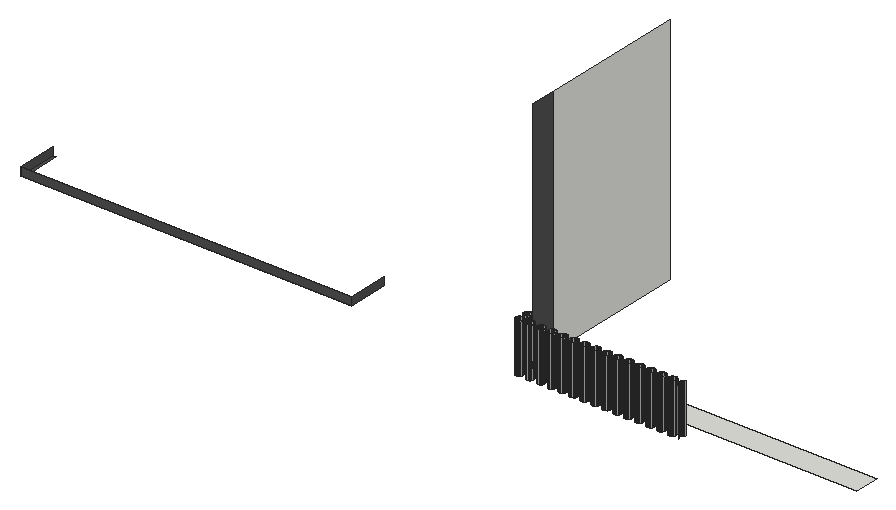
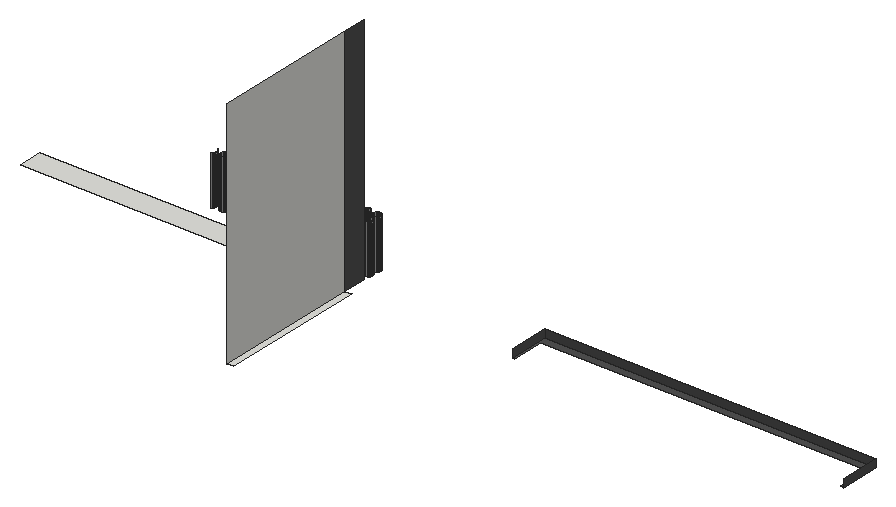
# SketchUp Ruby script. Lengths in inches.
U = 1.inch
M = Sketchup.active_model
def pt(a) = Geom::Point3d.new(a.map { |v| v * U })
def face(e, loops, mat)
  f = e.add_face(loops[0].map { |a| pt(a) })
  loops[1..].each { |l| e.add_face(l.map { |a| pt(a) }).erase! }
  f.material = f.back_material = mat if mat
  f
end
# faces: each face lists its corners as indices into pts; further lists are holes
def faces(e, pts, list, mat = nil) = list.each { |f| face(e, (f[0].is_a?(Array) ? f : [f]).map { |l| l.map { |i| pts[i] } }, mat) }
# xy, xz, yz: faces in a plane at the given z, y or x. An outline is a flat list of corners, or four numbers for a rectangle; further outlines are holes
def ring(l) = l.size == 4 ? [[l[0], l[1]], [l[2], l[1]], [l[2], l[3]], [l[0], l[3]]] : l.each_slice(2).to_a
def flat(e, list, mat, &to3) = list.each { |f| face(e, (f[0].is_a?(Array) ? f : [f]).map { |l| ring(l).map { |u, v| to3.(u, v) } }, mat) }
def xy(e, z, list, mat = nil) = flat(e, list, mat) { |x, y| [x, y, z] }
def xz(e, y, list, mat = nil) = flat(e, list, mat) { |x, z| [x, y, z] }
def yz(e, x, list, mat = nil) = flat(e, list, mat) { |y, z| [x, y, z] }
def lines(e, pts, list) = list.each { |a, b| e.add_line(pt(pts[a]), pt(pts[b])) }
# prism: a flat outline (further loops are holes) pulled along v
def prism(e, loops, v, mat = nil)
  f = face(e, loops, mat); d = Geom::Vector3d.new(v.map { |x| x * U })
  f.pushpull(f.normal.samedirection?(d) ? d.length : -d.length)
end
def box(e, o, s, mat = nil) = prism(e, [[o, [o[0] + s[0], o[1], o[2]], [o[0] + s[0], o[1] + s[1], o[2]], [o[0], o[1] + s[1], o[2]]]], [0, 0, s[2]], mat)
def at(x, y, z, deg = 0) = Geom::Transformation.translation(pt([x, y, z])) * Geom::Transformation.rotation(ORIGIN, Z_AXIS, deg.degrees)
def axes(o, x, y, z) = Geom::Transformation.new([*x, 0, *y, 0, *z, 0, *pt(o).to_a, 1])
def part(name) = M.definitions.add(name)
# library, detail: a bought-in or finely detailed component or shape, given as its bounding box
def library(name, o, s) = part(name).tap { |d| box(d.entities, o, s) }
def detail(e, o, s) = box(e.add_group.entities, o, s)
def put(e, d, t, mat = nil) = e.add_instance(d, t).tap { |i| i.material = mat if mat }
def group(e, t, mat = nil) = e.add_group.tap { |g| g.transformation = t; g.material = mat if mat }.entities
root = M.entities
M.materials.add("[0132_LightGray]").color = [169, 169, 169]
M.materials.add("[0135_DarkGray]").color = [81, 81, 81]
xy(root,180.23,[[54.57,34.6875,54.57,49.6875,55.95,49.6875,55.95,37.6875,176.89,37.6875,176.89,49.6875,177.76,49.6875,177.76,34.6875]],"[0135_DarkGray]")
xy(root,180.28,[[253.31,32.09,252.9375,32.13,252.59,32.28,252.29,32.51,252.0625,32.8,251.92,33.15,251.87,33.52,251.92,33.89,252.0625,34.24,252.29,34.54,252.59,34.77,252.9375,34.91,253.31,34.96,253.68,34.91,254.03,34.77,254.33,34.54,254.55,34.24,254.7,33.89,254.75,33.52,254.7,33.15,254.55,32.8,254.33,32.51,254.03,32.28,253.68,32.13],[257.37,32.09,257,32.13,256.65,32.28,256.35,32.51,256.125,32.8,255.98,33.15,255.93,33.52,255.98,33.89,256.125,34.24,256.35,34.54,256.65,34.77,257,34.91,257.37,34.96,257.74,34.91,258.09,34.77,258.39,34.54,258.62,34.24,258.76,33.89,258.81,33.52,258.76,33.15,258.62,32.8,258.39,32.51,258.09,32.28,257.74,32.13],[261.43,32.09,261.0625,32.13,260.72,32.28,260.42,32.51,260.1875,32.8,260.05,33.15,260,33.52,260.05,33.89,260.1875,34.24,260.42,34.54,260.72,34.77,261.0625,34.91,261.43,34.96,261.81,34.91,262.15,34.77,262.45,34.54,262.68,34.24,262.82,33.89,262.87,33.52,262.82,33.15,262.68,32.8,262.45,32.51,262.15,32.28,261.81,32.13],[265.5,32.09,265.125,32.13,264.78,32.28,264.48,32.51,264.25,32.8,264.11,33.15,264.06,33.52,264.11,33.89,264.25,34.24,264.48,34.54,264.78,34.77,265.125,34.91,265.5,34.96,265.87,34.91,266.22,34.77,266.51,34.54,266.74,34.24,266.88,33.89,266.93,33.52,266.88,33.15,266.74,32.8,266.51,32.51,266.22,32.28,265.87,32.13],[269.56,32.09,269.1875,32.13,268.84,32.28,268.54,32.51,268.3125,32.8,268.17,33.15,268.12,33.52,268.17,33.89,268.3125,34.24,268.54,34.54,268.84,34.77,269.1875,34.91,269.56,34.96,269.93,34.91,270.28,34.77,270.58,34.54,270.8,34.24,270.95,33.89,271,33.52,270.95,33.15,270.8,32.8,270.58,32.51,270.28,32.28,269.93,32.13],
  [273.62,32.09,273.25,32.13,272.9,32.28,272.6,32.51,272.375,32.8,272.23,33.15,272.18,33.52,272.23,33.89,272.375,34.24,272.6,34.54,272.9,34.77,273.25,34.91,273.62,34.96,273.99,34.91,274.34,34.77,274.64,34.54,274.87,34.24,275.01,33.89,275.06,33.52,275.01,33.15,274.87,32.8,274.64,32.51,274.34,32.28,273.99,32.13],[277.68,32.09,277.3125,32.13,276.97,32.28,276.67,32.51,276.4375,32.8,276.3,33.15,276.25,33.52,276.3,33.89,276.4375,34.24,276.67,34.54,276.97,34.77,277.3125,34.91,277.68,34.96,278.06,34.91,278.4,34.77,278.7,34.54,278.93,34.24,279.07,33.89,279.12,33.52,279.07,33.15,278.93,32.8,278.7,32.51,278.4,32.28,278.06,32.13],[281.75,32.09,281.375,32.13,281.03,32.28,280.73,32.51,280.5,32.8,280.36,33.15,280.31,33.52,280.36,33.89,280.5,34.24,280.73,34.54,281.03,34.77,281.375,34.91,281.75,34.96,282.12,34.91,282.47,34.77,282.76,34.54,282.99,34.24,283.13,33.89,283.18,33.52,283.13,33.15,282.99,32.8,282.76,32.51,282.47,32.28,282.12,32.13],[285.81,32.09,285.4375,32.13,285.09,32.28,284.79,32.51,284.5625,32.8,284.42,33.15,284.37,33.52,284.42,33.89,284.5625,34.24,284.79,34.54,285.09,34.77,285.4375,34.91,285.81,34.96,286.18,34.91,286.53,34.77,286.83,34.54,287.05,34.24,287.2,33.89,287.25,33.52,287.2,33.15,287.05,32.8,286.83,32.51,286.53,32.28,286.18,32.13],[289.87,32.09,289.5,32.13,289.15,32.28,288.85,32.51,288.625,32.8,288.48,33.15,288.43,33.52,288.48,33.89,288.625,34.24,288.85,34.54,289.15,34.77,289.5,34.91,289.87,34.96,290.24,34.91,290.59,34.77,290.89,34.54,291.12,34.24,291.26,33.89,291.31,33.52,291.26,33.15,291.12,32.8,290.89,32.51,290.59,32.28,290.24,32.13],
  [293.93,32.09,293.5625,32.13,293.22,32.28,292.92,32.51,292.6875,32.8,292.55,33.15,292.5,33.52,292.55,33.89,292.6875,34.24,292.92,34.54,293.22,34.77,293.5625,34.91,293.93,34.96,294.31,34.91,294.65,34.77,294.95,34.54,295.18,34.24,295.32,33.89,295.37,33.52,295.32,33.15,295.18,32.8,294.95,32.51,294.65,32.28,294.31,32.13],[298,32.09,297.625,32.13,297.28,32.28,296.98,32.51,296.75,32.8,296.61,33.15,296.56,33.52,296.61,33.89,296.75,34.24,296.98,34.54,297.28,34.77,297.625,34.91,298,34.96,298.37,34.91,298.72,34.77,299.01,34.54,299.24,34.24,299.38,33.89,299.43,33.52,299.38,33.15,299.24,32.8,299.01,32.51,298.72,32.28,298.37,32.13],[241.12,35.71,240.75,35.76,240.4,35.9,240.1,36.13,239.875,36.43,239.73,36.78,239.68,37.15,239.73,37.52,239.875,37.87,240.1,38.16,240.4,38.39,240.75,38.54,241.12,38.59,241.49,38.54,241.84,38.39,242.14,38.16,242.37,37.87,242.51,37.52,242.56,37.15,242.51,36.78,242.37,36.43,242.14,36.13,241.84,35.9,241.49,35.76],[240.45,40.6875,360.89,49.6875],[237.76,49.6875,240.45,104.375]])
xz(root,34.6875,[[54.57,180.23,177.76,183.1]],"[0135_DarkGray]")
yz(root,54.57,[[34.6875,180.23,49.6875,183.1]],"[0135_DarkGray]")
yz(root,177.76,[[34.6875,180.23,49.6875,183.1]],"[0135_DarkGray]")
yz(root,240.45,[[49.6875,180.28,104.375,266.7]])
yz(root,240.45,[[40.6875,180.28,49.6875,266.7]],"[0135_DarkGray]")
p = [[240.4,32.28,180.28],[240.75,32.13,180.28],[240.75,32.13,198.6],[240.4,32.28,198.6],[241.12,32.09,180.28],[241.12,32.09,198.6],
  [241.49,32.13,180.28],[241.49,32.13,198.6],[241.84,32.28,180.28],[241.84,32.28,198.6],[244.47,32.28,180.28],[244.8125,32.13,180.28],
  [244.8125,32.13,198.6],[244.47,32.28,198.6],[245.18,32.09,180.28],[245.18,32.09,198.6],[245.56,32.13,180.28],[245.56,32.13,198.6],
  [245.9,32.28,180.28],[245.9,32.28,198.6],[248.53,32.28,180.28],[248.875,32.13,180.28],[248.875,32.13,198.6],[248.53,32.28,198.6],
  [249.25,32.09,180.28],[249.25,32.09,198.6],[249.62,32.13,180.28],[249.62,32.13,198.6],[249.97,32.28,180.28],[249.97,32.28,198.6],
  [252.59,32.28,180.28],[252.9375,32.13,180.28],[252.9375,32.13,198.6],[252.59,32.28,198.6],[253.31,32.09,180.28],[253.31,32.09,198.6],
  [253.68,32.13,180.28],[253.68,32.13,198.6],[254.03,32.28,180.28],[254.03,32.28,198.6],[256.65,32.28,180.28],[257,32.13,180.28],
  [257,32.13,198.6],[256.65,32.28,198.6],[257.37,32.09,180.28],[257.37,32.09,198.6],[257.74,32.13,180.28],[257.74,32.13,198.6],
  [258.09,32.28,180.28],[258.09,32.28,198.6],[260.72,32.28,180.28],[261.0625,32.13,180.28],[261.0625,32.13,198.6],[260.72,32.28,198.6],
  [261.43,32.09,180.28],[261.43,32.09,198.6],[261.81,32.13,180.28],[261.81,32.13,198.6],[262.15,32.28,180.28],[262.15,32.28,198.6],
  [264.78,32.28,180.28],[265.125,32.13,180.28],[265.125,32.13,198.6],[264.78,32.28,198.6],[265.5,32.09,180.28],[265.5,32.09,198.6],
  [265.87,32.13,180.28],[265.87,32.13,198.6],[266.22,32.28,180.28],[266.22,32.28,198.6],[268.84,32.28,180.28],[269.1875,32.13,180.28],
  [269.1875,32.13,198.6],[268.84,32.28,198.6],[269.56,32.09,180.28],[269.56,32.09,198.6],[269.93,32.13,180.28],[269.93,32.13,198.6],
  [270.28,32.28,180.28],[270.28,32.28,198.6],[272.9,32.28,180.28],[273.25,32.13,180.28],[273.25,32.13,198.6],[272.9,32.28,198.6],
  [273.62,32.09,180.28],[273.62,32.09,198.6],[273.99,32.13,180.28],[273.99,32.13,198.6],[274.34,32.28,180.28],[274.34,32.28,198.6],
  [276.97,32.28,180.28],[277.3125,32.13,180.28],[277.3125,32.13,198.6],[276.97,32.28,198.6],[277.68,32.09,180.28],[277.68,32.09,198.6],
  [278.06,32.13,180.28],[278.06,32.13,198.6],[278.4,32.28,180.28],[278.4,32.28,198.6],[281.03,32.28,180.28],[281.375,32.13,180.28],
  [281.375,32.13,198.6],[281.03,32.28,198.6],[281.75,32.09,180.28],[281.75,32.09,198.6],[282.12,32.13,180.28],[282.12,32.13,198.6],
  [282.47,32.28,180.28],[282.47,32.28,198.6],[285.09,32.28,180.28],[285.4375,32.13,180.28],[285.4375,32.13,198.6],[285.09,32.28,198.6],
  [285.81,32.09,180.28],[285.81,32.09,198.6],[286.18,32.13,180.28],[286.18,32.13,198.6],[286.53,32.28,180.28],[286.53,32.28,198.6],
  [289.15,32.28,180.28],[289.5,32.13,180.28],[289.5,32.13,198.6],[289.15,32.28,198.6],[289.87,32.09,180.28],[289.87,32.09,198.6],
  [290.24,32.13,180.28],[290.24,32.13,198.6],[290.59,32.28,180.28],[290.59,32.28,198.6],[293.22,32.28,180.28],[293.5625,32.13,180.28],
  [293.5625,32.13,198.6],[293.22,32.28,198.6],[293.93,32.09,180.28],[293.93,32.09,198.6],[294.31,32.13,180.28],[294.31,32.13,198.6],
  [294.65,32.28,180.28],[294.65,32.28,198.6],[297.28,32.28,180.28],[297.625,32.13,180.28],[297.625,32.13,198.6],[297.28,32.28,198.6],
  [298,32.09,180.28],[298,32.09,198.6],[298.37,32.13,180.28],[298.37,32.13,198.6],[298.72,32.28,180.28],[298.72,32.28,198.6],
  [240.1,32.51,180.28],[240.1,32.51,198.6],[242.14,32.51,180.28],[242.14,32.51,198.6],[244.17,32.51,180.28],[244.17,32.51,198.6],
  [246.2,32.51,180.28],[246.2,32.51,198.6],[248.23,32.51,180.28],[248.23,32.51,198.6],[250.26,32.51,180.28],[250.26,32.51,198.6],
  [252.29,32.51,180.28],[252.29,32.51,198.6],[254.33,32.51,180.28],[254.33,32.51,198.6],[256.35,32.51,180.28],[256.35,32.51,198.6],
  [258.39,32.51,180.28],[258.39,32.51,198.6],[260.42,32.51,180.28],[260.42,32.51,198.6],[262.45,32.51,180.28],[262.45,32.51,198.6],
  [264.48,32.51,180.28],[264.48,32.51,198.6],[266.51,32.51,180.28],[266.51,32.51,198.6],[268.54,32.51,180.28],[268.54,32.51,198.6],
  [270.58,32.51,180.28],[270.58,32.51,198.6],[272.6,32.51,180.28],[272.6,32.51,198.6],[274.64,32.51,180.28],[274.64,32.51,198.6],
  [276.67,32.51,180.28],[276.67,32.51,198.6],[278.7,32.51,180.28],[278.7,32.51,198.6],[280.73,32.51,180.28],[280.73,32.51,198.6],
  [282.76,32.51,180.28],[282.76,32.51,198.6],[284.79,32.51,180.28],[284.79,32.51,198.6],[286.83,32.51,180.28],[286.83,32.51,198.6],
  [288.85,32.51,180.28],[288.85,32.51,198.6],[290.89,32.51,180.28],[290.89,32.51,198.6],[292.92,32.51,180.28],[292.92,32.51,198.6],
  [294.95,32.51,180.28],[294.95,32.51,198.6],[296.98,32.51,180.28],[296.98,32.51,198.6],[299.01,32.51,180.28],[299.01,32.51,198.6],
  [301.04,32.51,180.28],[301.34,32.28,180.28],[301.34,32.28,198.6],[301.04,32.51,198.6],[239.875,32.8,180.28],[239.875,32.8,198.6],
  [242.37,32.8,180.28],[242.37,32.8,198.6],[243.9375,32.8,180.28],[243.9375,32.8,198.6],[246.43,32.8,180.28],[246.43,32.8,198.6],
  [248,32.8,180.28],[248,32.8,198.6],[250.49,32.8,180.28],[250.49,32.8,198.6],[252.0625,32.8,180.28],[252.0625,32.8,198.6],
  [254.55,32.8,180.28],[254.55,32.8,198.6],[256.125,32.8,180.28],[256.125,32.8,198.6],[258.62,32.8,180.28],[258.62,32.8,198.6],
  [260.1875,32.8,180.28],[260.1875,32.8,198.6],[262.68,32.8,180.28],[262.68,32.8,198.6],[264.25,32.8,180.28],[264.25,32.8,198.6],
  [266.74,32.8,180.28],[266.74,32.8,198.6],[268.3125,32.8,180.28],[268.3125,32.8,198.6],[270.8,32.8,180.28],[270.8,32.8,198.6],
  [272.375,32.8,180.28],[272.375,32.8,198.6],[274.87,32.8,180.28],[274.87,32.8,198.6],[276.4375,32.8,180.28],[276.4375,32.8,198.6],
  [278.93,32.8,180.28],[278.93,32.8,198.6],[280.5,32.8,180.28],[280.5,32.8,198.6],[282.99,32.8,180.28],[282.99,32.8,198.6],
  [284.5625,32.8,180.28],[284.5625,32.8,198.6],[287.05,32.8,180.28],[287.05,32.8,198.6],[288.625,32.8,180.28],[288.625,32.8,198.6],
  [291.12,32.8,180.28],[291.12,32.8,198.6],[292.6875,32.8,180.28],[292.6875,32.8,198.6],[295.18,32.8,180.28],[295.18,32.8,198.6],
  [296.75,32.8,180.28],[296.75,32.8,198.6],[299.24,32.8,180.28],[299.24,32.8,198.6],[300.8125,32.8,180.28],[300.8125,32.8,198.6],
  [239.73,33.15,180.28],[239.73,33.15,198.6],[242.51,33.15,180.28],[242.51,33.15,198.6],[243.8,33.15,180.28],[243.8,33.15,198.6],
  [246.57,33.15,180.28],[246.57,33.15,198.6],[247.86,33.15,180.28],[247.86,33.15,198.6],[250.63,33.15,180.28],[250.63,33.15,198.6],
  [251.92,33.15,180.28],[251.92,33.15,198.6],[254.7,33.15,180.28],[254.7,33.15,198.6],[255.98,33.15,180.28],[255.98,33.15,198.6],
  [258.76,33.15,180.28],[258.76,33.15,198.6],[260.05,33.15,180.28],[260.05,33.15,198.6],[262.82,33.15,180.28],[262.82,33.15,198.6],
  [264.11,33.15,180.28],[264.11,33.15,198.6],[266.88,33.15,180.28],[266.88,33.15,198.6],[268.17,33.15,180.28],[268.17,33.15,198.6],
  [270.95,33.15,180.28],[270.95,33.15,198.6],[272.23,33.15,180.28],[272.23,33.15,198.6],[275.01,33.15,180.28],[275.01,33.15,198.6],
  [276.3,33.15,180.28],[276.3,33.15,198.6],[279.07,33.15,180.28],[279.07,33.15,198.6],[280.36,33.15,180.28],[280.36,33.15,198.6],
  [283.13,33.15,180.28],[283.13,33.15,198.6],[284.42,33.15,180.28],[284.42,33.15,198.6],[287.2,33.15,180.28],[287.2,33.15,198.6],
  [288.48,33.15,180.28],[288.48,33.15,198.6],[291.26,33.15,180.28],[291.26,33.15,198.6],[292.55,33.15,180.28],[292.55,33.15,198.6],
  [295.32,33.15,180.28],[295.32,33.15,198.6],[296.61,33.15,180.28],[296.61,33.15,198.6],[299.38,33.15,180.28],[299.38,33.15,198.6],
  [300.67,33.15,180.28],[300.67,33.15,198.6],[239.68,33.52,180.28],[239.68,33.52,198.6],[242.56,33.52,180.28],[242.56,33.52,198.6],
  [243.75,33.52,180.28],[243.75,33.52,198.6],[246.62,33.52,180.28],[246.62,33.52,198.6],[247.81,33.52,180.28],[247.81,33.52,198.6],
  [250.68,33.52,180.28],[250.68,33.52,198.6],[251.87,33.52,180.28],[251.87,33.52,198.6],[254.75,33.52,180.28],[254.75,33.52,198.6],
  [255.93,33.52,180.28],[255.93,33.52,198.6],[258.81,33.52,180.28],[258.81,33.52,198.6],[260,33.52,180.28],[260,33.52,198.6],
  [262.87,33.52,180.28],[262.87,33.52,198.6],[264.06,33.52,180.28],[264.06,33.52,198.6],[266.93,33.52,180.28],[266.93,33.52,198.6],
  [268.12,33.52,180.28],[268.12,33.52,198.6],[271,33.52,180.28],[271,33.52,198.6],[272.18,33.52,180.28],[272.18,33.52,198.6],
  [275.06,33.52,180.28],[275.06,33.52,198.6],[276.25,33.52,180.28],[276.25,33.52,198.6],[279.12,33.52,180.28],[279.12,33.52,198.6],
  [280.31,33.52,180.28],[280.31,33.52,198.6],[283.18,33.52,180.28],[283.18,33.52,198.6],[284.37,33.52,180.28],[284.37,33.52,198.6],
  [287.25,33.52,180.28],[287.25,33.52,198.6],[288.43,33.52,180.28],[288.43,33.52,198.6],[291.31,33.52,180.28],[291.31,33.52,198.6],
  [292.5,33.52,180.28],[292.5,33.52,198.6],[295.37,33.52,180.28],[295.37,33.52,198.6],[296.56,33.52,180.28],[296.56,33.52,198.6],
  [299.43,33.52,180.28],[299.43,33.52,198.6],[300.62,33.52,180.28],[300.62,33.52,198.6],[239.73,33.89,180.28],[239.73,33.89,198.6],
  [242.51,33.89,180.28],[242.51,33.89,198.6],[243.8,33.89,180.28],[243.8,33.89,198.6],[246.57,33.89,180.28],[246.57,33.89,198.6],
  [247.86,33.89,180.28],[247.86,33.89,198.6],[250.63,33.89,180.28],[250.63,33.89,198.6],[251.92,33.89,180.28],[251.92,33.89,198.6],
  [254.7,33.89,180.28],[254.7,33.89,198.6],[255.98,33.89,180.28],[255.98,33.89,198.6],[258.76,33.89,180.28],[258.76,33.89,198.6],
  [260.05,33.89,180.28],[260.05,33.89,198.6],[262.82,33.89,180.28],[262.82,33.89,198.6],[264.11,33.89,180.28],[264.11,33.89,198.6],
  [266.88,33.89,180.28],[266.88,33.89,198.6],[268.17,33.89,180.28],[268.17,33.89,198.6],[270.95,33.89,180.28],[270.95,33.89,198.6],
  [272.23,33.89,180.28],[272.23,33.89,198.6],[275.01,33.89,180.28],[275.01,33.89,198.6],[276.3,33.89,180.28],[276.3,33.89,198.6],
  [279.07,33.89,180.28],[279.07,33.89,198.6],[280.36,33.89,180.28],[280.36,33.89,198.6],[283.13,33.89,180.28],[283.13,33.89,198.6],
  [284.42,33.89,180.28],[284.42,33.89,198.6],[287.2,33.89,180.28],[287.2,33.89,198.6],[288.48,33.89,180.28],[288.48,33.89,198.6],
  [291.26,33.89,180.28],[291.26,33.89,198.6],[292.55,33.89,180.28],[292.55,33.89,198.6],[295.32,33.89,180.28],[295.32,33.89,198.6],
  [296.61,33.89,180.28],[296.61,33.89,198.6],[299.38,33.89,180.28],[299.38,33.89,198.6],[300.67,33.89,180.28],[300.67,33.89,198.6],
  [239.875,34.24,180.28],[239.875,34.24,198.6],[242.37,34.24,180.28],[242.37,34.24,198.6],[243.9375,34.24,180.28],[243.9375,34.24,198.6],
  [246.43,34.24,180.28],[246.43,34.24,198.6],[248,34.24,180.28],[248,34.24,198.6],[250.49,34.24,180.28],[250.49,34.24,198.6],
  [252.0625,34.24,180.28],[252.0625,34.24,198.6],[254.55,34.24,180.28],[254.55,34.24,198.6],[256.125,34.24,180.28],[256.125,34.24,198.6],
  [258.62,34.24,180.28],[258.62,34.24,198.6],[260.1875,34.24,180.28],[260.1875,34.24,198.6],[262.68,34.24,180.28],[262.68,34.24,198.6],
  [264.25,34.24,180.28],[264.25,34.24,198.6],[266.74,34.24,180.28],[266.74,34.24,198.6],[268.3125,34.24,180.28],[268.3125,34.24,198.6],
  [270.8,34.24,180.28],[270.8,34.24,198.6],[272.375,34.24,180.28],[272.375,34.24,198.6],[274.87,34.24,180.28],[274.87,34.24,198.6],
  [276.4375,34.24,180.28],[276.4375,34.24,198.6],[278.93,34.24,180.28],[278.93,34.24,198.6],[280.5,34.24,180.28],[280.5,34.24,198.6],
  [282.99,34.24,180.28],[282.99,34.24,198.6],[284.5625,34.24,180.28],[284.5625,34.24,198.6],[287.05,34.24,180.28],[287.05,34.24,198.6],
  [288.625,34.24,180.28],[288.625,34.24,198.6],[291.12,34.24,180.28],[291.12,34.24,198.6],[292.6875,34.24,180.28],[292.6875,34.24,198.6],
  [295.18,34.24,180.28],[295.18,34.24,198.6],[296.75,34.24,180.28],[296.75,34.24,198.6],[299.24,34.24,180.28],[299.24,34.24,198.6],
  [300.8125,34.24,180.28],[300.8125,34.24,198.6],[240.1,34.54,180.28],[240.1,34.54,198.6],[242.14,34.54,180.28],[242.14,34.54,198.6],
  [244.17,34.54,180.28],[244.17,34.54,198.6],[246.2,34.54,180.28],[246.2,34.54,198.6],[248.23,34.54,180.28],[248.23,34.54,198.6],
  [250.26,34.54,180.28],[250.26,34.54,198.6],[252.29,34.54,180.28],[252.29,34.54,198.6],[254.33,34.54,180.28],[254.33,34.54,198.6],
  [256.35,34.54,180.28],[256.35,34.54,198.6],[258.39,34.54,180.28],[258.39,34.54,198.6],[260.42,34.54,180.28],[260.42,34.54,198.6],
  [262.45,34.54,180.28],[262.45,34.54,198.6],[264.48,34.54,180.28],[264.48,34.54,198.6],[266.51,34.54,180.28],[266.51,34.54,198.6],
  [268.54,34.54,180.28],[268.54,34.54,198.6],[270.58,34.54,180.28],[270.58,34.54,198.6],[272.6,34.54,180.28],[272.6,34.54,198.6],
  [274.64,34.54,180.28],[274.64,34.54,198.6],[276.67,34.54,180.28],[276.67,34.54,198.6],[278.7,34.54,180.28],[278.7,34.54,198.6],
  [280.73,34.54,180.28],[280.73,34.54,198.6],[282.76,34.54,180.28],[282.76,34.54,198.6],[284.79,34.54,180.28],[284.79,34.54,198.6],
  [286.83,34.54,180.28],[286.83,34.54,198.6],[288.85,34.54,180.28],[288.85,34.54,198.6],[290.89,34.54,180.28],[290.89,34.54,198.6],
  [292.92,34.54,180.28],[292.92,34.54,198.6],[294.95,34.54,180.28],[294.95,34.54,198.6],[296.98,34.54,180.28],[296.98,34.54,198.6],
  [299.01,34.54,180.28],[299.01,34.54,198.6],[301.04,34.54,180.28],[301.04,34.54,198.6],[240.4,34.77,180.28],[240.4,34.77,198.6],
  [241.84,34.77,180.28],[241.84,34.77,198.6],[244.47,34.77,180.28],[244.47,34.77,198.6],[245.9,34.77,180.28],[245.9,34.77,198.6],
  [248.53,34.77,180.28],[248.53,34.77,198.6],[249.97,34.77,180.28],[249.97,34.77,198.6],[252.59,34.77,180.28],[252.59,34.77,198.6],
  [254.03,34.77,180.28],[254.03,34.77,198.6],[256.65,34.77,180.28],[256.65,34.77,198.6],[258.09,34.77,180.28],[258.09,34.77,198.6],
  [260.72,34.77,180.28],[260.72,34.77,198.6],[262.15,34.77,180.28],[262.15,34.77,198.6],[264.78,34.77,180.28],[264.78,34.77,198.6],
  [266.22,34.77,180.28],[266.22,34.77,198.6],[268.84,34.77,180.28],[268.84,34.77,198.6],[270.28,34.77,180.28],[270.28,34.77,198.6],
  [272.9,34.77,180.28],[272.9,34.77,198.6],[274.34,34.77,180.28],[274.34,34.77,198.6],[276.97,34.77,180.28],[276.97,34.77,198.6],
  [278.4,34.77,180.28],[278.4,34.77,198.6],[281.03,34.77,180.28],[281.03,34.77,198.6],[282.47,34.77,180.28],[282.47,34.77,198.6],
  [285.09,34.77,180.28],[285.09,34.77,198.6],[286.53,34.77,180.28],[286.53,34.77,198.6],[289.15,34.77,180.28],[289.15,34.77,198.6],
  [290.59,34.77,180.28],[290.59,34.77,198.6],[293.22,34.77,180.28],[293.22,34.77,198.6],[294.65,34.77,180.28],[294.65,34.77,198.6],
  [297.28,34.77,180.28],[297.28,34.77,198.6],[298.72,34.77,180.28],[298.72,34.77,198.6],[301.34,34.77,180.28],[301.34,34.77,198.6],
  [240.75,34.91,180.28],[240.75,34.91,198.6],[241.49,34.91,180.28],[241.49,34.91,198.6],[244.8125,34.91,180.28],[244.8125,34.91,198.6],
  [245.56,34.91,180.28],[245.56,34.91,198.6],[248.875,34.91,180.28],[248.875,34.91,198.6],[249.62,34.91,180.28],[249.62,34.91,198.6],
  [252.9375,34.91,180.28],[252.9375,34.91,198.6],[253.68,34.91,180.28],[253.68,34.91,198.6],[257,34.91,180.28],[257,34.91,198.6],
  [257.74,34.91,180.28],[257.74,34.91,198.6],[261.0625,34.91,180.28],[261.0625,34.91,198.6],[261.81,34.91,180.28],[261.81,34.91,198.6],
  [265.125,34.91,180.28],[265.125,34.91,198.6],[265.87,34.91,180.28],[265.87,34.91,198.6],[269.1875,34.91,180.28],[269.1875,34.91,198.6],
  [269.93,34.91,180.28],[269.93,34.91,198.6],[273.25,34.91,180.28],[273.25,34.91,198.6],[273.99,34.91,180.28],[273.99,34.91,198.6],
  [277.3125,34.91,180.28],[277.3125,34.91,198.6],[278.06,34.91,180.28],[278.06,34.91,198.6],[281.375,34.91,180.28],[281.375,34.91,198.6],
  [282.12,34.91,180.28],[282.12,34.91,198.6],[285.4375,34.91,180.28],[285.4375,34.91,198.6],[286.18,34.91,180.28],[286.18,34.91,198.6],
  [289.5,34.91,180.28],[289.5,34.91,198.6],[290.24,34.91,180.28],[290.24,34.91,198.6],[293.5625,34.91,180.28],[293.5625,34.91,198.6],
  [294.31,34.91,180.28],[294.31,34.91,198.6],[297.625,34.91,180.28],[297.625,34.91,198.6],[298.37,34.91,180.28],[298.37,34.91,198.6],
  [301.6875,34.91,180.28],[301.6875,34.91,198.6],[241.12,34.96,180.28],[241.12,34.96,198.6],[245.18,34.96,180.28],[245.18,34.96,198.6],
  [249.25,34.96,180.28],[249.25,34.96,198.6],[253.31,34.96,180.28],[253.31,34.96,198.6],[257.37,34.96,180.28],[257.37,34.96,198.6],
  [261.43,34.96,180.28],[261.43,34.96,198.6],[265.5,34.96,180.28],[265.5,34.96,198.6],[269.56,34.96,180.28],[269.56,34.96,198.6],
  [273.62,34.96,180.28],[273.62,34.96,198.6],[277.68,34.96,180.28],[277.68,34.96,198.6],[281.75,34.96,180.28],[281.75,34.96,198.6],
  [285.81,34.96,180.28],[285.81,34.96,198.6],[289.87,34.96,180.28],[289.87,34.96,198.6],[293.93,34.96,180.28],[293.93,34.96,198.6],
  [298,34.96,180.28],[298,34.96,198.6],[240.75,35.76,180.28],[241.12,35.71,180.28],[241.12,35.71,198.6],[240.75,35.76,198.6],
  [241.49,35.76,180.28],[241.49,35.76,198.6],[240.4,35.9,180.28],[240.4,35.9,198.6],[241.84,35.9,180.28],[241.84,35.9,198.6],
  [240.1,36.13,180.28],[240.1,36.13,198.6],[242.14,36.13,180.28],[242.14,36.13,198.6],[239.875,36.43,180.28],[239.875,36.43,198.6],
  [242.37,36.43,180.28],[242.37,36.43,198.6],[239.73,36.78,180.28],[239.73,36.78,198.6],[242.51,36.78,180.28],[242.51,36.78,198.6],
  [239.68,37.15,180.28],[239.68,37.15,198.6],[242.56,37.15,180.28],[242.56,37.15,198.6],[239.73,37.52,180.28],[239.73,37.52,198.6],
  [242.51,37.52,180.28],[242.51,37.52,198.6],[239.875,37.87,180.28],[239.875,37.87,198.6],[242.37,37.87,180.28],[242.37,37.87,198.6],
  [240.1,38.16,180.28],[240.1,38.16,198.6],[242.14,38.16,180.28],[242.14,38.16,198.6],[240.4,38.39,180.28],[240.4,38.39,198.6],
  [241.84,38.39,180.28],[241.84,38.39,198.6],[240.75,38.54,180.28],[240.75,38.54,198.6],[241.49,38.54,180.28],[241.49,38.54,198.6],
  [241.12,38.59,180.28],[241.12,38.59,198.6],[176.89,37.6875,183.1],[176.89,37.6875,180.23]]
faces(root,p,[[0,1,2,3],[1,4,5,2],[4,6,7,5],[6,8,9,7],[10,11,12,13],[11,14,15,12],[14,16,17,15],[16,18,19,17],
  [20,21,22,23],[21,24,25,22],[24,26,27,25],[26,28,29,27],[30,31,32,33],[31,34,35,32],[34,36,37,35],[36,38,39,37],
  [40,41,42,43],[41,44,45,42],[44,46,47,45],[46,48,49,47],[50,51,52,53],[51,54,55,52],[54,56,57,55],[56,58,59,57],
  [60,61,62,63],[61,64,65,62],[64,66,67,65],[66,68,69,67],[70,71,72,73],[71,74,75,72],[74,76,77,75],[76,78,79,77],
  [80,81,82,83],[81,84,85,82],[84,86,87,85],[86,88,89,87],[90,91,92,93],[91,94,95,92],[94,96,97,95],[96,98,99,97],
  [100,101,102,103],[101,104,105,102],[104,106,107,105],[106,108,109,107],[110,111,112,113],[111,114,115,112],[114,116,117,115],[116,118,119,117],
  [120,121,122,123],[121,124,125,122],[124,126,127,125],[126,128,129,127],[130,131,132,133],[131,134,135,132],[134,136,137,135],[136,138,139,137],
  [140,141,142,143],[141,144,145,142],[144,146,147,145],[146,148,149,147],[150,0,3,151],[8,152,153,9],[154,10,13,155],[18,156,157,19],
  [158,20,23,159],[28,160,161,29],[162,30,33,163],[38,164,165,39],[166,40,43,167],[48,168,169,49],[170,50,53,171],[58,172,173,59],
  [174,60,63,175],[68,176,177,69],[178,70,73,179],[78,180,181,79],[182,80,83,183],[88,184,185,89],[186,90,93,187],[98,188,189,99],
  [190,100,103,191],[108,192,193,109],[194,110,113,195],[118,196,197,119],[198,120,123,199],[128,200,201,129],[202,130,133,203],[138,204,205,139],
  [206,140,143,207],[148,208,209,149],[210,211,212,213],[214,150,151,215],[152,216,217,153],[218,154,155,219],[156,220,221,157],[222,158,159,223],
  [160,224,225,161],[226,162,163,227],[164,228,229,165],[230,166,167,231],[168,232,233,169],[234,170,171,235],[172,236,237,173],[238,174,175,239],
  [176,240,241,177],[242,178,179,243],[180,244,245,181],[246,182,183,247],[184,248,249,185],[250,186,187,251],[188,252,253,189],[254,190,191,255],
  [192,256,257,193],[258,194,195,259],[196,260,261,197],[262,198,199,263],[200,264,265,201],[266,202,203,267],[204,268,269,205],[270,206,207,271],
  [208,272,273,209],[274,210,213,275],[276,214,215,277],[216,278,279,217],[280,218,219,281],[220,282,283,221],[284,222,223,285],[224,286,287,225],
  [288,226,227,289],[228,290,291,229],[292,230,231,293],[232,294,295,233],[296,234,235,297],[236,298,299,237],[300,238,239,301],[240,302,303,241],
  [304,242,243,305],[244,306,307,245],[308,246,247,309],[248,310,311,249],[312,250,251,313],[252,314,315,253],[316,254,255,317],[256,318,319,257],
  [320,258,259,321],[260,322,323,261],[324,262,263,325],[264,326,327,265],[328,266,267,329],[268,330,331,269],[332,270,271,333],[272,334,335,273],
  [336,274,275,337],[338,276,277,339],[278,340,341,279],[342,280,281,343],[282,344,345,283],[346,284,285,347],[286,348,349,287],[350,288,289,351],
  [290,352,353,291],[354,292,293,355],[294,356,357,295],[358,296,297,359],[298,360,361,299],[362,300,301,363],[302,364,365,303],[366,304,305,367],
  [306,368,369,307],[370,308,309,371],[310,372,373,311],[374,312,313,375],[314,376,377,315],[378,316,317,379],[318,380,381,319],[382,320,321,383],
  [322,384,385,323],[386,324,325,387],[326,388,389,327],[390,328,329,391],[330,392,393,331],[394,332,333,395],[334,396,397,335],[398,336,337,399],
  [400,338,339,401],[340,402,403,341],[404,342,343,405],[344,406,407,345],[408,346,347,409],[348,410,411,349],[412,350,351,413],[352,414,415,353],
  [416,354,355,417],[356,418,419,357],[420,358,359,421],[360,422,423,361],[424,362,363,425],[364,426,427,365],[428,366,367,429],[368,430,431,369],
  [432,370,371,433],[372,434,435,373],[436,374,375,437],[376,438,439,377],[440,378,379,441],[380,442,443,381],[444,382,383,445],[384,446,447,385],
  [448,386,387,449],[388,450,451,389],[452,390,391,453],[392,454,455,393],[456,394,395,457],[396,458,459,397],[460,398,399,461],[462,400,401,463],
  [402,464,465,403],[466,404,405,467],[406,468,469,407],[470,408,409,471],[410,472,473,411],[474,412,413,475],[414,476,477,415],[478,416,417,479],
  [418,480,481,419],[482,420,421,483],[422,484,485,423],[486,424,425,487],[426,488,489,427],[490,428,429,491],[430,492,493,431],[494,432,433,495],
  [434,496,497,435],[498,436,437,499],[438,500,501,439],[502,440,441,503],[442,504,505,443],[506,444,445,507],[446,508,509,447],[510,448,449,511],
  [450,512,513,451],[514,452,453,515],[454,516,517,455],[518,456,457,519],[458,520,521,459],[522,460,461,523],[524,462,463,525],[464,526,527,465],
  [528,466,467,529],[468,530,531,469],[532,470,471,533],[472,534,535,473],[536,474,475,537],[476,538,539,477],[540,478,479,541],[480,542,543,481],
  [544,482,483,545],[484,546,547,485],[548,486,487,549],[488,550,551,489],[552,490,491,553],[492,554,555,493],[556,494,495,557],[496,558,559,497],
  [560,498,499,561],[500,562,563,501],[564,502,503,565],[504,566,567,505],[568,506,507,569],[508,570,571,509],[572,510,511,573],[512,574,575,513],
  [576,514,515,577],[516,578,579,517],[580,518,519,581],[520,582,583,521],[584,522,523,585],[586,524,525,587],[526,588,589,527],[590,528,529,591],
  [530,592,593,531],[594,532,533,595],[534,596,597,535],[598,536,537,599],[538,600,601,539],[602,540,541,603],[542,604,605,543],[606,544,545,607],
  [546,608,609,547],[610,548,549,611],[550,612,613,551],[614,552,553,615],[554,616,617,555],[618,556,557,619],[558,620,621,559],[622,560,561,623],
  [562,624,625,563],[626,564,565,627],[566,628,629,567],[630,568,569,631],[570,632,633,571],[634,572,573,635],[574,636,637,575],[638,576,577,639],
  [578,640,641,579],[642,580,581,643],[582,644,645,583],[646,584,585,647],[648,586,587,649],[588,650,651,589],[652,590,591,653],[592,654,655,593],
  [656,594,595,657],[596,658,659,597],[660,598,599,661],[600,662,663,601],[664,602,603,665],[604,666,667,605],[668,606,607,669],[608,670,671,609],
  [672,610,611,673],[612,674,675,613],[676,614,615,677],[616,678,679,617],[680,618,619,681],[620,682,683,621],[684,622,623,685],[624,686,687,625],
  [688,626,627,689],[628,690,691,629],[692,630,631,693],[632,694,695,633],[696,634,635,697],[636,698,699,637],[700,638,639,701],[640,702,703,641],
  [704,642,643,705],[644,706,707,645],[708,646,647,709],[710,648,649,711],[650,710,711,651],[712,652,653,713],[654,712,713,655],[714,656,657,715],
  [658,714,715,659],[716,660,661,717],[662,716,717,663],[718,664,665,719],[666,718,719,667],[720,668,669,721],[670,720,721,671],[722,672,673,723],
  [674,722,723,675],[724,676,677,725],[678,724,725,679],[726,680,681,727],[682,726,727,683],[728,684,685,729],[686,728,729,687],[730,688,689,731],
  [690,730,731,691],[732,692,693,733],[694,732,733,695],[734,696,697,735],[698,734,735,699],[736,700,701,737],[702,736,737,703],[738,704,705,739],
  [706,738,739,707],[740,741,742,743],[741,744,745,742],[746,740,743,747],[744,748,749,745],[750,746,747,751],[748,752,753,749],[754,750,751,755],
  [752,756,757,753],[758,754,755,759],[756,760,761,757],[762,758,759,763],[760,764,765,761],[766,762,763,767],[764,768,769,765],[770,766,767,771],
  [768,772,773,769],[774,770,771,775],[772,776,777,773],[778,774,775,779],[776,780,781,777],[782,778,779,783],[780,784,785,781],[786,782,783,787],
  [784,786,787,785]],"[0132_LightGray]")
lines(root,p,[[788,789]])
